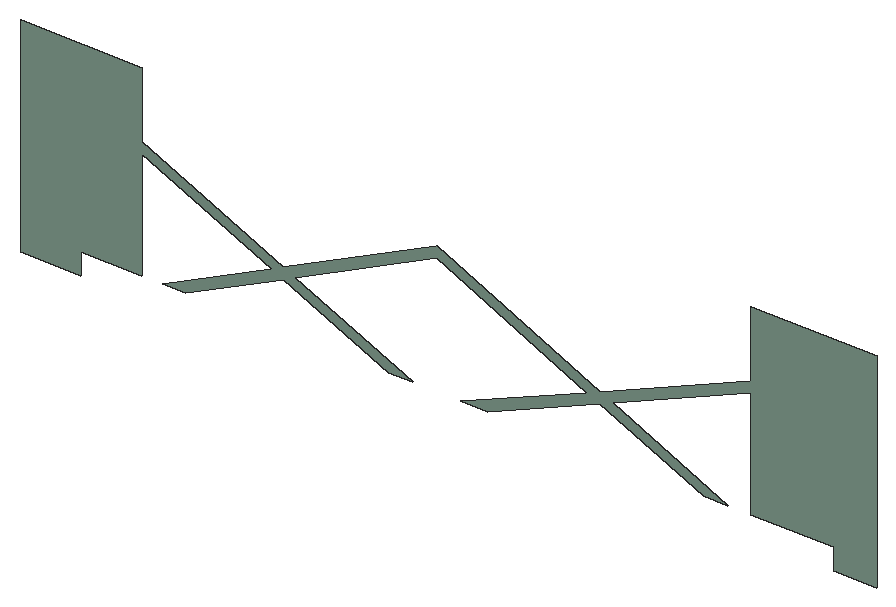
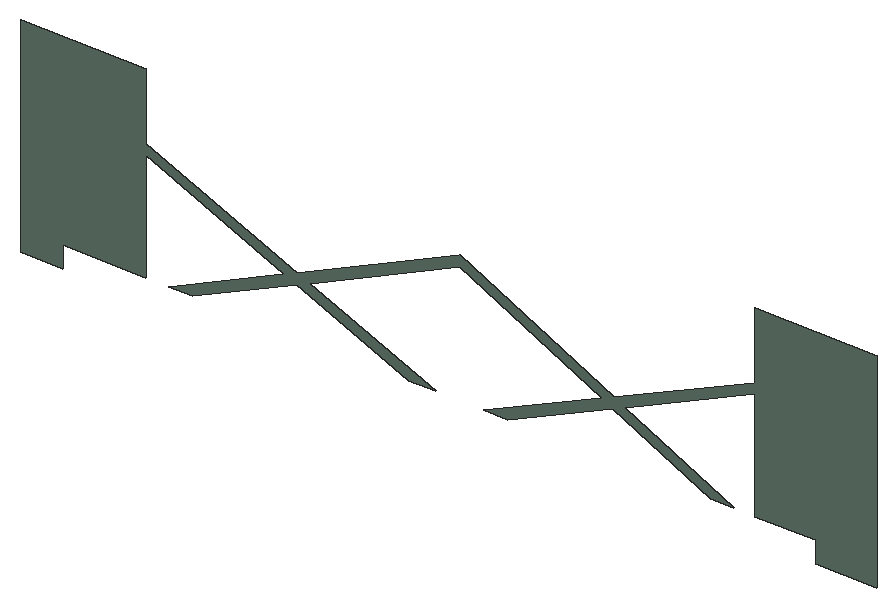
# SketchUp Ruby script. Lengths in inches.
U = 1.inch
M = Sketchup.active_model
def pt(a) = Geom::Point3d.new(a.map { |v| v * U })
def face(e, loops, mat)
  f = e.add_face(loops[0].map { |a| pt(a) })
  loops[1..].each { |l| e.add_face(l.map { |a| pt(a) }).erase! }
  f.material = f.back_material = mat if mat
  f
end
# faces: each face lists its corners as indices into pts; further lists are holes
def faces(e, pts, list, mat = nil) = list.each { |f| face(e, (f[0].is_a?(Array) ? f : [f]).map { |l| l.map { |i| pts[i] } }, mat) }
# xy, xz, yz: faces in a plane at the given z, y or x. An outline is a flat list of corners, or four numbers for a rectangle; further outlines are holes
def ring(l) = l.size == 4 ? [[l[0], l[1]], [l[2], l[1]], [l[2], l[3]], [l[0], l[3]]] : l.each_slice(2).to_a
def flat(e, list, mat, &to3) = list.each { |f| face(e, (f[0].is_a?(Array) ? f : [f]).map { |l| ring(l).map { |u, v| to3.(u, v) } }, mat) }
def xy(e, z, list, mat = nil) = flat(e, list, mat) { |x, y| [x, y, z] }
def xz(e, y, list, mat = nil) = flat(e, list, mat) { |x, z| [x, y, z] }
def yz(e, x, list, mat = nil) = flat(e, list, mat) { |y, z| [x, y, z] }
def lines(e, pts, list) = list.each { |a, b| e.add_line(pt(pts[a]), pt(pts[b])) }
# prism: a flat outline (further loops are holes) pulled along v
def prism(e, loops, v, mat = nil)
  f = face(e, loops, mat); d = Geom::Vector3d.new(v.map { |x| x * U })
  f.pushpull(f.normal.samedirection?(d) ? d.length : -d.length)
end
def box(e, o, s, mat = nil) = prism(e, [[o, [o[0] + s[0], o[1], o[2]], [o[0] + s[0], o[1] + s[1], o[2]], [o[0], o[1] + s[1], o[2]]]], [0, 0, s[2]], mat)
def at(x, y, z, deg = 0) = Geom::Transformation.translation(pt([x, y, z])) * Geom::Transformation.rotation(ORIGIN, Z_AXIS, deg.degrees)
def axes(o, x, y, z) = Geom::Transformation.new([*x, 0, *y, 0, *z, 0, *pt(o).to_a, 1])
def part(name) = M.definitions.add(name)
# library, detail: a bought-in or finely detailed component or shape, given as its bounding box
def library(name, o, s) = part(name).tap { |d| box(d.entities, o, s) }
def detail(e, o, s) = box(e.add_group.entities, o, s)
def put(e, d, t, mat = nil) = e.add_instance(d, t).tap { |i| i.material = mat if mat }
def group(e, t, mat = nil) = e.add_group.tap { |g| g.transformation = t; g.material = mat if mat }.entities
root = M.entities
M.materials.add("[Color H08]").color = [130, 158, 143]
xz(root,85.1875,[[0,9,21.01,9,21.01,16.375,42.01,16.375,42.01,54.29,86.99,34.34,49.44,16.375,57.43,16.375,91.13,32.5,127.49,16.375,135.91,16.375,95.125,34.41,144.11,57.85,196.33,34.44,152.53,16.375,161.86,16.375,200.67,32.5,236.65,16.375,245.17,16.375,205.09,34.34,253.1,54.29,253.1,16.375,281.76,16.375,281.76,9,296.4375,9,296.4375,81,253.1,81,253.1,57.86,200.77,36.27,144.11,61.67,90.97,36.24,42.01,57.9,42.01,81,0,81]],"[Color H08]")
